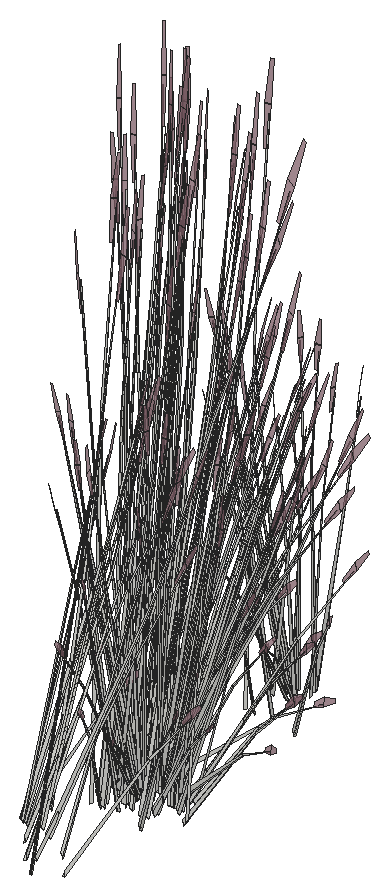
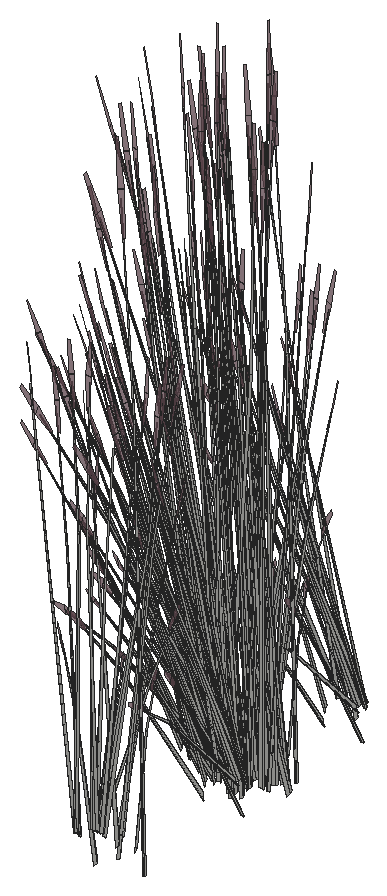
# SketchUp Ruby script. Lengths in inches.
U = 1.inch
M = Sketchup.active_model
def pt(a) = Geom::Point3d.new(a.map { |v| v * U })
def face(e, loops, mat)
  f = e.add_face(loops[0].map { |a| pt(a) })
  loops[1..].each { |l| e.add_face(l.map { |a| pt(a) }).erase! }
  f.material = f.back_material = mat if mat
  f
end
# faces: each face lists its corners as indices into pts; further lists are holes
def faces(e, pts, list, mat = nil) = list.each { |f| face(e, (f[0].is_a?(Array) ? f : [f]).map { |l| l.map { |i| pts[i] } }, mat) }
# xy, xz, yz: faces in a plane at the given z, y or x. An outline is a flat list of corners, or four numbers for a rectangle; further outlines are holes
def ring(l) = l.size == 4 ? [[l[0], l[1]], [l[2], l[1]], [l[2], l[3]], [l[0], l[3]]] : l.each_slice(2).to_a
def flat(e, list, mat, &to3) = list.each { |f| face(e, (f[0].is_a?(Array) ? f : [f]).map { |l| ring(l).map { |u, v| to3.(u, v) } }, mat) }
def xy(e, z, list, mat = nil) = flat(e, list, mat) { |x, y| [x, y, z] }
def xz(e, y, list, mat = nil) = flat(e, list, mat) { |x, z| [x, y, z] }
def yz(e, x, list, mat = nil) = flat(e, list, mat) { |y, z| [x, y, z] }
def lines(e, pts, list) = list.each { |a, b| e.add_line(pt(pts[a]), pt(pts[b])) }
# prism: a flat outline (further loops are holes) pulled along v
def prism(e, loops, v, mat = nil)
  f = face(e, loops, mat); d = Geom::Vector3d.new(v.map { |x| x * U })
  f.pushpull(f.normal.samedirection?(d) ? d.length : -d.length)
end
def box(e, o, s, mat = nil) = prism(e, [[o, [o[0] + s[0], o[1], o[2]], [o[0] + s[0], o[1] + s[1], o[2]], [o[0], o[1] + s[1], o[2]]]], [0, 0, s[2]], mat)
def at(x, y, z, deg = 0) = Geom::Transformation.translation(pt([x, y, z])) * Geom::Transformation.rotation(ORIGIN, Z_AXIS, deg.degrees)
def axes(o, x, y, z) = Geom::Transformation.new([*x, 0, *y, 0, *z, 0, *pt(o).to_a, 1])
def part(name) = M.definitions.add(name)
# library, detail: a bought-in or finely detailed component or shape, given as its bounding box
def library(name, o, s) = part(name).tap { |d| box(d.entities, o, s) }
def detail(e, o, s) = box(e.add_group.entities, o, s)
def put(e, d, t, mat = nil) = e.add_instance(d, t).tap { |i| i.material = mat if mat }
def group(e, t, mat = nil) = e.add_group.tap { |g| g.transformation = t; g.material = mat if mat }.entities
root = M.entities
M.materials.add("LightPink_Translucent").color = [144, 107, 117]
M.materials["LightPink_Translucent"].alpha = 0.75
c1 = part("blade")
p = [[2.15,0.21,22],[0,0.17,0],[0.09,0.45,0],[2.18,0.31,22],[2.29,0.31,22],[0.38,0.45,0],
  [2.48,0.24,33],[2.49,0.24,33],[2.48,0.22,33]]
faces(c1.entities,p,[[0,1,2,3],[4,5,2,3],[6,3,4,7],[8,0,3,6]])
c2 = part("seeds")
p = [[0.3,-0.1,1.38],[-0.01,-0.03,1.59],[-0.01,-0.03,0.03],[0.14,-0.07,-0.07],[0.29,-0.03,3],[0.15,0.01,3.11]]
faces(c2.entities,p,[[0,1,2,3],[1,0,4,5]],"LightPink_Translucent")
c3 = part("blade with seeds")
put(c3.entities,c1,at(0,0,0))
put(c3.entities,c2,axes([2.4,0.25,30.99],[1.5799,-0.05474,1.17369],[-0.12525,1.92788,0.29478],[-0.07173,-0.02425,1.56792]))
put(root,c3,axes([347.41,137.86,3.79],[0.06518,-0.0942,1.76342],[0.82057,-0.27742,-0.26939],[0.24877,0.14358,0.30037]))
put(root,c3,axes([346.33,135.72,4.39],[0.32803,0.59738,-0.69212],[-0.94492,0.21515,-0.18165],[0.03626,0.20229,1.52773]))
put(root,c3,axes([346.13,137.42,6.97],[0.88277,-0.1551,-0.51099],[0.15442,0.58737,-0.3958],[0.23711,0.16832,0.97773]))
put(root,c3,axes([343.68,137.51,7.34],[0.2697,-0.50175,0.35414],[0.78684,0.14635,-0.4572],[0.07215,0.20201,0.87481]))
put(root,c3,axes([347.35,138.02,4.96],[-0.57368,-0.02046,1.0506],[0.37886,-0.43461,0.58006],[0.22663,0.15441,0.8241]))
put(root,c3,axes([345.7,137.91,7.02],[-0.4066,0.41448,0.0643],[-0.57901,-0.24131,0.50621],[0.18719,0.13288,0.77189]))
put(root,c3,axes([344.74,139.3,7.9375],[0.61821,-0.37431,-0.06488],[0.56645,0.40995,-0.29416],[0.03988,0.11616,0.97024]))
put(root,c3,axes([345.87,137.79,7.03],[-0.88979,0.14973,0.48003],[-0.15442,-0.58737,0.3958],[0.20926,0.17311,0.9933]))
put(root,c3,axes([345.48,136.97,4.88],[0.01579,-0.21629,1.43002],[0.75442,-0.24159,-0.30754],[0.23289,0.25887,0.61141]))
put(root,c3,axes([346.1,146.48,4.88],[-0.25429,0.13207,1.43002],[-0.76157,-0.23115,-0.30754],[0.14117,-0.28747,0.61141]))
put(root,c3,axes([343.42,137.72,7.33],[0.87543,-0.30377,-0.1216],[0.4302,0.53915,-0.67495],[0.1155,0.2272,1.02557]))
put(root,c3,axes([343.58,137.84,3.79],[0.14478,-0.0355,1.76342],[0.8709,0.19542,-0.26939],[0.02547,0.22025,0.30037]))
put(root,c3,axes([346.72,147.46,7.27],[0.02328,-0.60353,-0.71045],[0.98022,0.04053,0.08574],[0.10344,-0.25568,1.00501]))
put(root,c3,axes([348.09,146.52,7.01],[-0.00864,-0.12985,1.74944],[-0.72937,-0.3753,-0.27667],[0.11277,-0.2275,0.14031]))
put(root,c3,axes([344.17,137.7,6.97],[0.87941,0.16356,-0.51099],[-0.30143,0.56078,-0.3958],[0.08064,0.22578,0.97773]))
put(root,c3,axes([345.62,147.15,6.17],[-0.16657,0.22426,1.71376],[-0.69879,-0.4641,0.13857],[0.31524,-0.28926,0.73262]))
put(root,c3,axes([347.89,146.05,7],[-0.09085,0.04984,1.77383],[-0.89014,-0.16814,-0.16761],[-0.03222,-0.21748,0.31391]))
put(root,c3,axes([344.67,136.54,6.17],[-0.2045,-0.20949,1.71376],[0.94495,-0.17636,0.13857],[0.21357,0.32887,0.73262]))
put(root,c3,axes([343.77,138.04,6.82],[-0.2697,0.50175,-0.35414],[-0.78684,-0.14635,0.4572],[0.07215,0.20201,0.87481]))
put(root,c3,axes([345.16,145.43,5.06],[0.11476,0.38047,1.1486],[-0.63664,-0.21072,0.84392],[0.06851,-0.19481,0.25299]))
put(root,c3,axes([346.52,147.26,6.97],[-0.64041,-0.4384,-0.51099],[0.67652,-0.38394,-0.3958],[0.09744,-0.22274,0.97773]))
put(root,c3,axes([345.12,146.61,7.03],[0.88151,0.17057,0.48003],[-0.30143,0.56078,0.3958],[-0.05297,-0.22053,0.9933]))
put(root,c3,axes([347.19,147.49,7.33],[-0.98321,-0.03233,-0.1216],[0.02687,-0.61208,-0.67495],[0.0683,-0.23574,1.02557]))
put(root,c3,axes([343.85,137.59,7.27],[0.42698,0.53052,-0.71045],[-0.87893,0.29566,0.08574],[0.09984,0.25633,1.00501]))
put(root,c3,axes([347.12,147.1,6.82],[0.60531,-0.34352,-0.35414],[0.573,0.39225,0.4572],[0.08718,-0.19929,0.87481]))
put(root,c3,axes([345.35,146.56,7.02],[0.6592,-0.22175,0.0643],[0.32265,0.40436,0.50621],[-0.06366,-0.17825,0.77189]))
put(root,c3,axes([343.21,138.93,7.01],[0.1134,0.10507,1.74944],[0.91515,0.04128,-0.27667],[0.09203,0.23172,0.14031]))
put(root,c3,axes([347.88,146.89,3.79],[-0.1339,-0.0514,1.76342],[-0.34394,-0.57425,-0.26939],[0.23202,-0.15583,0.30037]))
put(root,c3,axes([347.12,147.23,7.03],[0.63704,0.44518,0.48003],[-0.67652,0.38394,0.3958],[0.11751,-0.20886,0.9933]))
put(root,c3,axes([347.36,147.27,7.02],[0.73517,0.0304,0.0643],[-0.02016,0.45906,0.50621],[0.07693,-0.17585,0.77189]))
put(root,c3,axes([346.81,147.58,7.34],[-0.60531,0.34352,0.35414],[-0.573,-0.39225,-0.4572],[0.08718,-0.19929,0.87481]))
put(root,c3,axes([347.875,148.51,7.27],[0.4673,-0.51481,-0.71045],[0.81887,0.36587,0.08574],[0.27902,-0.18652,1.00501]))
put(root,c3,axes([342.82,147.01,4.67],[-0.55932,-0.6538,0],[0.93577,-0.36461,-0.51607],[0.21313,-0.08304,1.63711]))
put(root,c3,axes([347.85,148.27,6.97],[-0.22982,-0.59576,-0.51099],[0.87033,-0.10422,-0.3958],[0.24941,-0.16002,0.97773]))
put(root,c3,axes([348.26,148.7,7.33],[-0.82753,-0.35977,-0.1216],[0.47675,-0.52101,-0.67495],[0.2338,-0.18111,1.02557]))
put(root,c3,axes([343.58,146.91,4.3125],[0.83726,-0.32623,-0.49651],[0.50045,0.58498,0],[0.19069,-0.0743,1.57504]))
put(root,c3,axes([348.55,148.04,4.88],[-0.31959,-0.01933,1.43002],[-0.32741,-0.51843,-0.30754],[0.39262,-0.14666,0.61141]))
put(root,c3,axes([350.3,148.54,7],[-0.11685,-0.00496,1.77383],[-0.48522,-0.53096,-0.16761],[0.19486,-0.17458,0.31391]))
put(root,c3,axes([344.57,148.25,4.35],[0.60257,-0.49041,-0.62353],[0.74854,0.44469,-0.16365],[0.24146,-0.12234,1.37633]))
put(root,c3,axes([348.92,147.08,5.06],[-0.29798,0.33213,1.1486],[-0.25612,-0.44624,0.84392],[0.24611,-0.11182,0.25299]))
put(root,c3,axes([348.49,148.33,6.82],[0.77872,-0.09325,-0.35414],[0.20563,0.53305,0.4572],[0.22316,-0.14318,0.87481]))
put(root,c3,axes([343.53,149.11,4.5],[0.43405,-0.58792,-0.44739],[0.90188,0.28295,0.21531],[0,-0.13553,1.43643]))
put(root,c3,axes([343.92,148.82,4.96],[-0.10425,-0.7445,-0.29095],[1.08575,-0.04502,-0.50002],[0.19119,-0.09917,1.59708]))
put(root,c3,axes([347.86,148.65,7.34],[-0.77872,0.09325,0.35414],[-0.20563,-0.53305,-0.4572],[0.22316,-0.14318,0.87481]))
put(root,c3,axes([343.78,147.17,4.32],[0.83462,0.16144,-0.30978],[-0.21015,0.56852,0.30978],[0.16826,-0.06556,1.38974]))
put(root,c3,axes([348.5625,148.5625,7.02],[0.61415,0.2744,0.0643],[-0.35756,0.39076,0.50621],[0.1969,-0.12633,0.77189]))
put(root,c3,axes([348.39,148.45,7.03],[0.22187,0.60049,0.48003],[-0.87033,0.10422,0.3958],[0.25651,-0.14123,0.9933]))
put(root,c3,axes([350.74,149.17,7.01],[0.12414,-0.09938,1.74944],[-0.15889,-0.60963,-0.27667],[0.31148,-0.11559,0.14031]))
put(root,c3,axes([344.0625,149.4,4.73],[1.00799,0.31623,0.24065],[-0.48511,0.65709,0.50002],[0,-0.15147,1.60543]))
put(root,c3,axes([343.74,148.96,5.01],[-0.97146,0.04028,0.44739],[-0.08785,-0.66859,-0.21531],[0.17391,-0.06776,1.43643]))
put(root,c3,axes([348.29,150.1,7.33],[-0.45012,-0.59081,-0.1216],[0.79888,-0.29033,-0.67495],[0.33665,-0.07795,1.02557]))
put(root,c3,axes([348.26,149.59,6.97],[0.24236,-0.59349,-0.51099],[0.83094,0.20343,-0.3958],[0.33455,-0.05442,0.97773]))
put(root,c3,axes([346.94,147.18,4.67],[0.55932,-0.6538,0],[0.93577,0.36461,-0.51607],[0.21313,0.08304,1.63711]))
put(root,c3,axes([349.14,149.76,4.28],[-0.57619,0.0783,1.41583],[-0.09171,-0.62326,0.08104],[0.40356,-0.09434,0.80566]))
put(root,c3,axes([350.19,149.21,4.55],[-0.55463,-0.41721,-0.06488],[0.60744,-0.38228,-0.29416],[0.17212,-0.02691,0.97024]))
put(root,c3,axes([345.1,149.26,4.5],[0,-0.75495,0],[1.11865,0,0],[0,0,1.79456]))
put(root,c3,axes([346.46,147.52,4.77],[-0.83726,-0.32623,0.49651],[0.50045,-0.58498,0],[0.19069,0.0743,1.57504]))
put(root,c3,axes([348.1,149.81,7.27],[0.78611,-0.28816,-0.71045],[0.4381,0.59317,0.08574],[0.37982,-0.06738,1.00501]))
put(root,c3,axes([344.57,148.79,4.65],[-0.74176,0.59212,0.45755],[-0.88124,-0.52269,0.17955],[0.17882,-0.05909,1.58856]))
put(root,c3,axes([343.29,147.8125,4.77],[-0.25843,0.64844,0.17642],[-0.9457,-0.1835,0.35086],[0.16336,-0.00316,1.60407]))
put(root,c3,axes([347.98,149.92,7.34],[-0.74348,-0.18202,0.35414],[0.21685,-0.53102,-0.4572],[0.29933,-0.04869,0.87481]))
put(root,c3,axes([342.89,148.33,3.89],[-0.88056,0.26122,1.28929],[-0.28027,-0.74951,0.50096],[0.54072,0.01247,1.46642]))
put(root,c3,axes([345.26,148.53,4.91],[0.17258,-0.58229,0.1448],[0.84319,0.10108,-0.41347],[0.15345,0.05979,1.26744]))
put(root,c3,axes([349.77,149.35,3.79],[-0.04675,-0.09906,1.76342],[0.32428,-0.57943,-0.26939],[0.32711,-0.00833,0.30037]))
put(root,c3,axes([344.9,148.68,5.01],[-0.53742,-0.54764,0.44739],[0.81403,-0.38564,-0.21531],[0.17391,0.06776,1.43643]))
put(root,c3,axes([345.17,148.72,4.96],[0.90324,-0.43318,-0.29095],[0.60064,0.61207,-0.50002],[0.22285,0.06216,1.59708]))
put(root,c3,axes([348.76,149.86,6.82],[0.74348,0.18202,-0.35414],[-0.21685,0.53102,0.4572],[0.29933,-0.04869,0.87481]))
put(root,c3,axes([347.45,147.57,4.3125],[0.83726,0.32623,-0.49651],[-0.50045,0.58498,0],[0.19069,0.0743,1.57504]))
put(root,c3,axes([345.86,149.43,4.5],[1.00089,0,0],[0,0.67548,0],[0,0,1.78407]))
put(root,c3,axes([346.15,147.85,4.77],[-0.96132,0.17317,0.17642],[-0.23737,-0.64447,0.35086],[0.08574,0.0939,1.60407]))
put(root,c3,axes([346.74,149.21,6.17],[-0.37107,0.01478,1.71376],[0.24616,-0.64047,0.13857],[0.5288,0.03961,0.73262]))
put(root,c3,axes([347.22,147.8125,4.32],[0.21015,0.56852,-0.30978],[-0.83462,0.16144,0.30978],[0.16826,0.06556,1.38974]))
put(root,c3,axes([348.66,150.09,7.02],[0.32857,0.44488,0.0643],[-0.59916,0.21775,0.50621],[0.26412,-0.04296,0.77189]))
put(root,c3,axes([345.54,149.09,4.67],[-1.13071,-0.13747,0.49198],[0.23011,-0.77639,0.19306],[0.16524,0.07497,1.70813]))
put(root,c3,axes([348.59,149.93,7.03],[-0.25275,0.59491,0.48003],[-0.83094,-0.20343,0.3958],[0.32677,-0.03575,0.9933]))
put(root,c3,axes([344.64,151,4.5],[-0.29189,-0.56252,0],[0.83351,-0.19699,0],[0,0,1.54371]))
put(root,c3,axes([345.73,150.92,4.48],[0.93921,-0.22138,-0.19198],[0.33003,0.6377,0.00008],[0.10367,-0.02447,1.73897]))
put(root,c3,axes([345.84,149.72,4.51],[0.62448,0.42144,0],[-0.62448,0.42144,0],[0,0,1.69266]))
put(root,c3,axes([347.53,149.54,4.77],[-0.70288,-0.47526,0.17642],[0.70832,-0.46097,0.35086],[-0.07763,0.09706,1.60407]))
put(root,c3,axes([346.23,148.82,4.35],[0.9306,0.10697,-0.62353],[-0.19638,0.65984,-0.16365],[0.27771,0.07995,1.37633]))
put(root,c3,axes([350.34,149.97,5.06],[-0.55274,0.10771,1.1486],[0.26018,-0.44517,0.84392],[0.29323,0.03046,0.25299]))
put(root,c3,axes([345.83,149.23,5.01],[0.43405,-0.58792,0.44739],[0.90188,0.28295,-0.21531],[0,0.13553,1.43643]))
put(root,c3,axes([350.09,151.85,7],[-0.08089,-0.05712,1.77383],[0.17695,-0.61228,-0.16761],[0.31864,-0.03912,0.31391]))
put(root,c3,axes([345.67,149.5625,4.59],[0,0.75458,-0.05637],[-1.11865,0,0],[0,0.02371,1.79368]))
put(root,c3,axes([345.75,149.03,4.5],[0.53742,0.54764,-0.44739],[-0.81403,0.38564,0.21531],[0.17391,0.06776,1.43643]))
put(root,c3,axes([349.38,151.34,6.22],[-0.17122,-0.54847,-0.03492],[0.80929,-0.12609,-0.15832],[0.169,0.03477,0.52218]))
put(root,c3,axes([347.28,151.33,7.33],[0.0479,-0.66354,-0.1216],[0.90696,0.01814,-0.67495],[0.3493,0.04609,1.02557]))
put(root,c3,axes([348.11,149.55,4.77],[0,-0.65246,0.49651],[1.00089,0,0],[0,0.1486,1.57504]))
put(root,c3,axes([346.21,149.36,4.91],[0.83351,-0.19028,0.1448],[0.29189,0.54335,-0.41347],[0,0.11958,1.26744]))
put(root,c3,axes([347.14,151.07,7.34],[-0.50902,-0.40851,0.35414],[0.58122,-0.38671,-0.4572],[0.29531,0.05884,0.87481]))
put(root,c3,axes([349.31,150.69,4.88],[-0.21545,-0.16047,1.43002],[0.28033,-0.53085,-0.30754],[0.43591,0.07191,0.61141]))
put(root,c3,axes([345.45,151.27,4.5],[0.90188,0.29293,0],[-0.43405,0.60866,0],[0,0,1.74954]))
put(root,c3,axes([348.07,150.93,7.01],[0.19191,-0.01103,1.74944],[0.52639,-0.5069,-0.27667],[0.34136,0.06691,0.14031]))
put(root,c3,axes([347.33,151.01,7.27],[0.89428,0.01571,-0.71045],[-0.06006,0.66153,0.08574],[0.37886,0.06981,1.00501]))
put(root,c3,axes([345.13,151.02,4.58],[0.38895,0.74956,-0.06012],[-1.11135,0.26265,0],[0.01358,0.02618,1.72173]))
put(root,c3,axes([348.79,149.67,4.67],[1.11865,0,0],[0,0.72922,-0.51607],[0,0.16609,1.63711]))
put(root,c3,axes([348.34,150.04,4.49],[-1.1181,-0.00522,-0.04976],[0,-0.72922,0.49943],[-0.03514,0.166,1.58352]))
put(root,c3,axes([345.92,149.41,4.96],[1.00749,0.31132,-0.29095],[-0.48511,0.65709,-0.50002],[0.03166,0.16133,1.59708]))
put(root,c3,axes([347.87,151.28,6.82],[0.50902,0.40851,-0.35414],[-0.58122,0.38671,0.4572],[0.29531,0.05884,0.87481]))
put(root,c3,axes([348.11,150.15,4.32],[-0.62448,0.40708,-0.30978],[-0.62448,-0.40708,0.30978],[0,0.13112,1.38974]))
put(root,c3,axes([347.61,151.4375,7.02],[-0.04505,0.49615,0.0643],[-0.68022,-0.0136,0.50621],[0.26056,0.05192,0.77189]))
put(root,c3,axes([345.81,149.89,4.5],[-0.43405,0.58792,-0.44739],[-0.90188,-0.28295,0.21531],[0,0.13553,1.43643]))
put(root,c3,axes([347.67,151.28,7.03],[-0.65964,0.42992,0.48003],[-0.5689,-0.45657,0.3958],[0.30948,0.0793,0.9933]))
put(root,c3,axes([345.57,151.78,7.34],[-0.13817,-0.52554,0.35414],[0.78985,-0.13877,-0.4572],[0.21215,0.1506,0.87481]))
put(root,c3,axes([348.54,150.16,4.3125],[0,0.65246,-0.49651],[-1.00089,0,0],[0,0.1486,1.57504]))
put(root,c3,axes([346.04,150.23,6.17],[-0.3323,-0.11241,1.71376],[0.68769,-0.4716,0.13857],[0.42861,0.21275,0.73262]))
put(root,c3,axes([346.1,148.75,6.77],[-0.77304,-0.33901,1.38283],[0.81626,-0.52782,0.59665],[0.24941,0.31809,1.33663]))
put(root,c3,axes([347.27,151.51,5.06],[-0.5037,-0.18761,1.1486],[0.6504,-0.19062,0.84392],[0.17543,0.16147,0.25299]))
put(root,c3,axes([345.5,152.05,7.33],[0.53309,-0.55848,-0.1216],[0.77201,0.32175,-0.67495],[0.26836,0.15779,1.02557]))
put(root,c3,axes([344.8,152.51,7],[0.00265,-0.07899,1.77383],[0.76665,-0.34851,-0.16761],[0.2663,0.12439,0.31391]))
put(root,c3,axes([347.41,152.21,3.79],[0.06518,-0.0942,1.76342],[0.82057,-0.27742,-0.26939],[0.24877,0.14358,0.30037]))
put(root,c3,axes([346.33,150.07,4.39],[0.32803,0.59738,-0.69212],[-0.94492,0.21515,-0.18165],[0.03626,0.20229,1.52773]))
put(root,c3,axes([346.13,151.77,6.97],[0.88277,-0.1551,-0.51099],[0.15442,0.58737,-0.3958],[0.23711,0.16832,0.97773]))
put(root,c3,axes([343.68,151.86,7.34],[0.2697,-0.50175,0.35414],[0.78684,0.14635,-0.4572],[0.07215,0.20201,0.87481]))
put(root,c3,axes([347.35,152.37,4.96],[-0.57368,-0.02046,1.0506],[0.37886,-0.43461,0.58006],[0.22663,0.15441,0.8241]))
put(root,c3,axes([345.7,152.25,7.02],[-0.4066,0.41448,0.0643],[-0.57901,-0.24131,0.50621],[0.18719,0.13288,0.77189]))
put(root,c3,axes([344.74,153.65,7.9375],[0.61821,-0.37431,-0.06488],[0.56645,0.40995,-0.29416],[0.03988,0.11616,0.97024]))
put(root,c3,axes([345.87,152.14,7.03],[-0.88979,0.14973,0.48003],[-0.15442,-0.58737,0.3958],[0.20926,0.17311,0.9933]))
put(root,c3,axes([345.48,151.3125,4.88],[0.01579,-0.21629,1.43002],[0.75442,-0.24159,-0.30754],[0.23289,0.25887,0.61141]))
put(root,c3,axes([343.42,152.07,7.33],[0.87543,-0.30377,-0.1216],[0.4302,0.53915,-0.67495],[0.1155,0.2272,1.02557]))
put(root,c3,axes([343.58,152.19,3.79],[0.14478,-0.0355,1.76342],[0.8709,0.19542,-0.26939],[0.02547,0.22025,0.30037]))
put(root,c3,axes([344.17,152.04,6.97],[0.87941,0.16356,-0.51099],[-0.30143,0.56078,-0.3958],[0.08064,0.22578,0.97773]))
put(root,c3,axes([344.67,150.89,6.17],[-0.2045,-0.20949,1.71376],[0.94495,-0.17636,0.13857],[0.21357,0.32887,0.73262]))
put(root,c3,axes([343.77,152.39,6.82],[-0.2697,0.50175,-0.35414],[-0.78684,-0.14635,0.4572],[0.07215,0.20201,0.87481]))
put(root,c3,axes([343.85,151.9375,7.27],[0.42698,0.53052,-0.71045],[-0.87893,0.29566,0.08574],[0.09984,0.25633,1.00501]))
put(root,c3,axes([343.21,153.28,7.01],[0.1134,0.10507,1.74944],[0.91515,0.04128,-0.27667],[0.09203,0.23172,0.14031]))
put(root,c3,axes([346.1,164.65,4.88],[-0.25429,0.13207,1.43002],[-0.76157,-0.23115,-0.30754],[0.14117,-0.28747,0.61141]))
put(root,c3,axes([346.72,165.625,7.27],[0.02328,-0.60353,-0.71045],[0.98022,0.04053,0.08574],[0.10344,-0.25568,1.00501]))
put(root,c3,axes([348.09,164.68,7.01],[-0.00864,-0.12985,1.74944],[-0.72937,-0.3753,-0.27667],[0.11277,-0.2275,0.14031]))
put(root,c3,axes([345.62,165.32,6.17],[-0.16657,0.22426,1.71376],[-0.69879,-0.4641,0.13857],[0.31524,-0.28926,0.73262]))
put(root,c3,axes([347.89,164.22,7],[-0.09085,0.04984,1.77383],[-0.89014,-0.16814,-0.16761],[-0.03222,-0.21748,0.31391]))
put(root,c3,axes([345.16,163.6,5.06],[0.11476,0.38047,1.1486],[-0.63664,-0.21072,0.84392],[0.06851,-0.19481,0.25299]))
put(root,c3,axes([346.52,165.42,6.97],[-0.64041,-0.4384,-0.51099],[0.67652,-0.38394,-0.3958],[0.09744,-0.22274,0.97773]))
put(root,c3,axes([345.12,164.77,7.03],[0.88151,0.17057,0.48003],[-0.30143,0.56078,0.3958],[-0.05297,-0.22053,0.9933]))
put(root,c3,axes([347.19,165.66,7.33],[-0.98321,-0.03233,-0.1216],[0.02687,-0.61208,-0.67495],[0.0683,-0.23574,1.02557]))
put(root,c3,axes([347.12,165.26,6.82],[0.60531,-0.34352,-0.35414],[0.573,0.39225,0.4572],[0.08718,-0.19929,0.87481]))
put(root,c3,axes([345.35,164.73,7.02],[0.6592,-0.22175,0.0643],[0.32265,0.40436,0.50621],[-0.06366,-0.17825,0.77189]))
put(root,c3,axes([347.88,165.05,3.79],[-0.1339,-0.0514,1.76342],[-0.34394,-0.57425,-0.26939],[0.23202,-0.15583,0.30037]))
put(root,c3,axes([347.12,165.4,7.03],[0.63704,0.44518,0.48003],[-0.67652,0.38394,0.3958],[0.11751,-0.20886,0.9933]))
put(root,c3,axes([347.36,165.4375,7.02],[0.73517,0.0304,0.0643],[-0.02016,0.45906,0.50621],[0.07693,-0.17585,0.77189]))
put(root,c3,axes([346.81,165.75,7.34],[-0.60531,0.34352,0.35414],[-0.573,-0.39225,-0.4572],[0.08718,-0.19929,0.87481]))
put(root,c3,axes([347.875,166.67,7.27],[0.4673,-0.51481,-0.71045],[0.81887,0.36587,0.08574],[0.27902,-0.18652,1.00501]))
put(root,c3,axes([342.82,165.18,4.67],[-0.55932,-0.6538,0],[0.93577,-0.36461,-0.51607],[0.21313,-0.08304,1.63711]))
put(root,c3,axes([347.85,166.43,6.97],[-0.22982,-0.59576,-0.51099],[0.87033,-0.10422,-0.3958],[0.24941,-0.16002,0.97773]))
put(root,c3,axes([348.26,166.86,7.33],[-0.82753,-0.35977,-0.1216],[0.47675,-0.52101,-0.67495],[0.2338,-0.18111,1.02557]))
